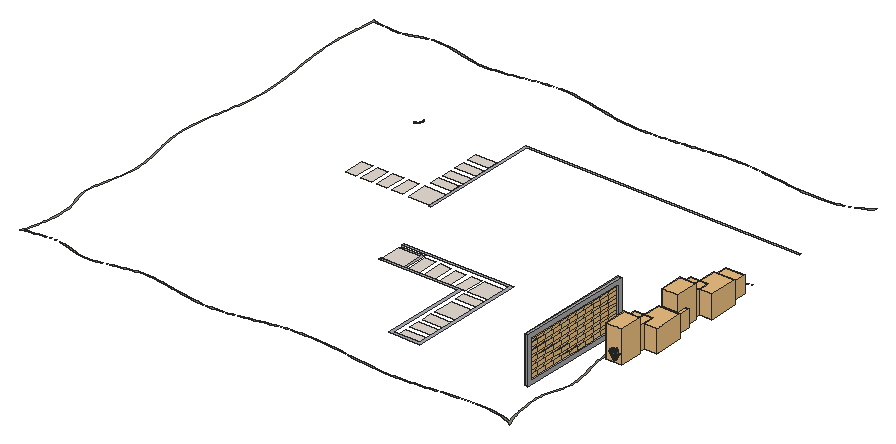
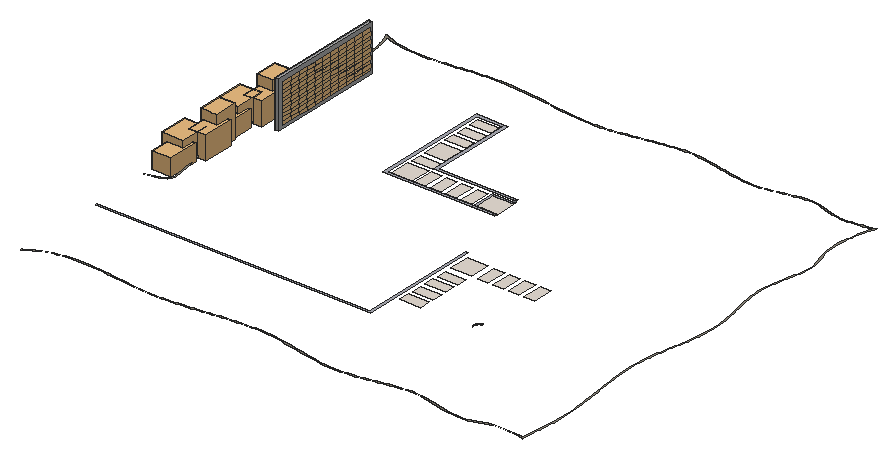
# SketchUp Ruby script. Lengths in inches.
U = 1.inch
M = Sketchup.active_model
def pt(a) = Geom::Point3d.new(a.map { |v| v * U })
def face(e, loops, mat)
  f = e.add_face(loops[0].map { |a| pt(a) })
  loops[1..].each { |l| e.add_face(l.map { |a| pt(a) }).erase! }
  f.material = f.back_material = mat if mat
  f
end
# faces: each face lists its corners as indices into pts; further lists are holes
def faces(e, pts, list, mat = nil) = list.each { |f| face(e, (f[0].is_a?(Array) ? f : [f]).map { |l| l.map { |i| pts[i] } }, mat) }
# xy, xz, yz: faces in a plane at the given z, y or x. An outline is a flat list of corners, or four numbers for a rectangle; further outlines are holes
def ring(l) = l.size == 4 ? [[l[0], l[1]], [l[2], l[1]], [l[2], l[3]], [l[0], l[3]]] : l.each_slice(2).to_a
def flat(e, list, mat, &to3) = list.each { |f| face(e, (f[0].is_a?(Array) ? f : [f]).map { |l| ring(l).map { |u, v| to3.(u, v) } }, mat) }
def xy(e, z, list, mat = nil) = flat(e, list, mat) { |x, y| [x, y, z] }
def xz(e, y, list, mat = nil) = flat(e, list, mat) { |x, z| [x, y, z] }
def yz(e, x, list, mat = nil) = flat(e, list, mat) { |y, z| [x, y, z] }
def lines(e, pts, list) = list.each { |a, b| e.add_line(pt(pts[a]), pt(pts[b])) }
# prism: a flat outline (further loops are holes) pulled along v
def prism(e, loops, v, mat = nil)
  f = face(e, loops, mat); d = Geom::Vector3d.new(v.map { |x| x * U })
  f.pushpull(f.normal.samedirection?(d) ? d.length : -d.length)
end
def box(e, o, s, mat = nil) = prism(e, [[o, [o[0] + s[0], o[1], o[2]], [o[0] + s[0], o[1] + s[1], o[2]], [o[0], o[1] + s[1], o[2]]]], [0, 0, s[2]], mat)
def at(x, y, z, deg = 0) = Geom::Transformation.translation(pt([x, y, z])) * Geom::Transformation.rotation(ORIGIN, Z_AXIS, deg.degrees)
def axes(o, x, y, z) = Geom::Transformation.new([*x, 0, *y, 0, *z, 0, *pt(o).to_a, 1])
def part(name) = M.definitions.add(name)
# library, detail: a bought-in or finely detailed component or shape, given as its bounding box
def library(name, o, s) = part(name).tap { |d| box(d.entities, o, s) }
def detail(e, o, s) = box(e.add_group.entities, o, s)
def put(e, d, t, mat = nil) = e.add_instance(d, t).tap { |i| i.material = mat if mat }
def group(e, t, mat = nil) = e.add_group.tap { |g| g.transformation = t; g.material = mat if mat }.entities
root = M.entities
M.materials.add("M03_Pewter_Shine").color = [168, 168, 168]
M.materials.add("Marble_01_1K").color = [230, 221, 211]
M.materials.add("Marble_07_1K").color = [36, 34, 36]
M.materials.add("Marble_20_1K").color = [172, 173, 182]
M.materials.add("Material__4").color = [36, 36, 36]
M.materials.add("Material__6").color = [79, 108, 5]
M.materials.add("Plaster_06_1K").color = [141, 135, 122]
M.materials.add("calathea lutea").color = [121, 145, 80]
c1 = library("Group\#103",[-0.1,0,0],[4.88,24.05,8.12])
c2 = part("Timber rail")
put(c2.entities,c1,axes([5.13,208.76,0],[-1,0,0],[0,-0.96445,0],[0,0,1]))
put(c2.entities,c1,axes([4.82,46.39,0],[-1,0,0],[0,-0.96445,0],[0,0,1]))
put(c2.entities,c1,axes([5,139.17,0],[-1,0,0],[0,-0.96445,0],[0,0,1]))
put(c2.entities,c1,axes([5.09,185.5625,0],[-1,0,0],[0,-0.96445,0],[0,0,1]))
put(c2.entities,c1,axes([5.04,162.37,0],[-1,0,0],[0,-0.96445,0],[0,0,1]))
put(c2.entities,c1,axes([4.87,69.59,0],[-1,0,0],[0,-0.96445,0],[0,0,1]))
put(c2.entities,c1,axes([4.95,115.98,0],[-1,0,0],[0,-0.96445,0],[0,0,1]))
put(c2.entities,c1,axes([5.18,231.95,0],[-1,0,0],[0,-0.96445,0],[0,0,1]))
put(c2.entities,c1,axes([4.91,92.78,0],[-1,0,0],[0,-0.96445,0],[0,0,1]))
put(c2.entities,c1,axes([4.78,23.2,0],[-1,0,0],[0,-0.96445,0],[0,0,1]))
put(c2.entities,c1,axes([5.22,255.15,0],[-1,0,0],[0,-0.96445,0],[0,0,1]))
c3 = library("Group\#105",[0,0,0],[4.875,24.05,8.12])
c4 = part("Group\#104")
put(c4.entities,c3,axes([4.875,240.5,0],[-1,0,0],[0,1,0],[0,0,1]))
put(c4.entities,c3,axes([6.32,0,0],[-1,0,0],[0,1,0],[0,0,1]))
put(c4.entities,c3,axes([5.45,144.3,0],[-1,0,0],[0,1,0],[0,0,1]))
put(c4.entities,c3,axes([5.31,168.35,0],[-1,0,0],[0,1,0],[0,0,1]))
put(c4.entities,c3,axes([5.6,120.25,0],[-1,0,0],[0,1,0],[0,0,1]))
put(c4.entities,c3,axes([6.03,48.1,0],[-1,0,0],[0,1,0],[0,0,1]))
put(c4.entities,c3,axes([5.74,96.2,0],[-1,0,0],[0,1,0],[0,0,1]))
put(c4.entities,c3,axes([5.89,72.15,0],[-1,0,0],[0,1,0],[0,0,1]))
put(c4.entities,c3,axes([6.18,24.05,0],[-1,0,0],[0,1,0],[0,0,1]))
put(c4.entities,c3,axes([5.17,192.4,0],[-1,0,0],[0,1,0],[0,0,1]))
put(c4.entities,c3,axes([5.02,216.45,0],[-1,0,0],[0,1,0],[0,0,1]))
c5 = part("Group\#156")
g1 = group(c5.entities,at(8.61,38.85,0))
xy(g1,0,[[0,0,2.82,19.1,22.58,0],[22.58,0,2.82,19.1,22.58,19.1]],"calathea lutea")
p = [[2.82,19.1,0],[7.19,48.22,5.13],[10.77,48.22,5.13],[12.74,48.22,5.13],[22.58,48.22,5.13],[22.58,19.1,0]]
faces(g1,p,[[0,1,2,3,4,5]],"calathea lutea")
g2 = group(c5.entities,at(-0.77,-7.77,0))
p = [[14.8125,23.31,1.46],[21.35,23.31,0],[14.8125,0,1.46],[21.35,0,0],[27.89,0,1.46],[27.89,23.31,1.46],
  [8.27,46.62,2.92],[21.35,46.62,0],[34.4375,46.62,2.92],[4.47,23.31,6.43],[0,0,8.59],[33.76,0,4.28],
  [33.76,23.31,4.28]]
faces(g2,p,[[0,1,2],[3,2,1],[4,3,5],[1,5,3],[6,7,0],[1,0,7],[5,1,8],[7,8,1],
  [9,0,2,10],[11,4,5,12],[9,6,0],[12,5,8]],"calathea lutea")
c6 = part("Group\#150")
xy(c6.entities,0,[[0,0,0,33.87,27.21,33.87,19.71,0]],"calathea lutea")
c7 = part("Group\#157")
xy(c7.entities,1.04,[[21.13,33.87,21.13,57.59,32.375,57.59,27.12,33.87]],"calathea lutea")
xy(c7.entities,1.32,[[0.12,33.87,7.74,57.59]],"calathea lutea")
p = [[7.74,33.87,1.32],[11.8,57.59,0.61],[15.24,57.59,0],[15.24,33.87,0],[18.43,57.59,0.5625],[21.13,57.59,1.04],
  [21.13,33.87,1.04],[15.24,77.7,2.36],[21.13,77.7,3.4],[7.74,57.59,1.32],[7.74,77.7,3.69],[36.83,77.7,3.4],
  [32.375,57.59,1.04],[0.12,57.59,1.32],[0.12,77.7,3.69]]
faces(c7.entities,p,[[0,1,2,3],[3,2,4],[3,4,5,6],[7,2,1],[8,4,2,7],[0,9,1],[7,1,9,10],[8,5,4],
  [11,12,5,8],[10,9,13,14]],"calathea lutea")
put(c7.entities,c6,axes([0,-16.9375,0],[1,0,0],[0,1.5,0],[0,0,1]))
c8 = part("Group\#155")
g3 = group(c8.entities,at(0,-17.3,0))
xy(g3,0,[[0,0,28.07,51.9]],"calathea lutea")
g4 = group(c8.entities,at(0.9,34.6,0))
xy(g4,0,[[13.14,0,13.14,26.22,16.85,26.22],[13.14,0,16.85,26.22,20.16,26.22,20.16,0]],"calathea lutea")
p = [[6.36,0,1.82],[9.95,26.22,0.86],[13.14,26.22,0],[13.14,0,0],[20.16,0,0],[20.16,26.22,0],
  [27.07,26.22,1.22],[27.07,0,1.22],[13.14,49.5625,5.91],[20.16,49.5625,5.91],[16.85,26.22,0],[27.07,49.5625,7.125],
  [6.36,26.22,1.82],[6.36,49.5625,7.72],[0,0,4.78],[0,26.22,4.78],[0,49.5625,10.6875]]
faces(g4,p,[[0,1,2,3],[4,5,6,7],[8,2,1],[9,10,2,8],[9,5,10],[11,6,5,9],[0,12,1],[8,1,12,13],
  [14,15,12,0],[13,12,15,16]],"calathea lutea")
c9 = part("Group\#154")
put(c9.entities,c6,axes([0,-16.9375,0],[1,0,0],[0,1.5,0],[0,0,1]))
g5 = group(c9.entities,at(-0.23,33.4,-0.35))
p = [[15.12,39.14,-19.87],[15.12,20.54,-11.86],[11.68,20.84,-11.33],[21.02,39.66,-18.97],[18.3125,20.82,-11.37],[7.62,21.2,-10.71],
  [7.62,39.8,-18.72],[21.02,21.06,-10.96],[36.72,39.66,-18.97],[32.26,21.06,-10.96],[0,21.2,-10.71],[0,39.8,-18.72],
  [7.62,0.66,1.15],[15.12,0,0],[21.02,0.52,0.9],[27.01,0.52,0.9],[0,0.66,1.15]]
faces(g5,p,[[0,1,2],[3,4,1,0],[0,2,5,6],[3,7,4],[8,9,7,3],[6,5,10,11],[12,2,1,13],[13,1,4],
  [13,4,7,14],[12,5,2],[14,7,9,15],[16,10,5,12]],"calathea lutea")
c10 = part("Foliage cluster")
put(c10.entities,c5,axes([37.24,8.07,75.17],[1,0,0],[0,0.45554,-0.89021],[0,0.89021,0.45554]))
put(c10.entities,c7,axes([69.44,65.48,16.68],[-0.53288,-0.84619,0],[0.14694,-0.09253,0.98481],[-0.83334,0.52478,0.17365]))
put(c10.entities,c8,axes([47.9375,70.43,17.04],[0.74664,-0.66523,0],[0.11552,0.12965,0.98481],[-0.65512,-0.7353,0.17365]))
put(c10.entities,c5,axes([76.19,10.66,75.17],[0.70711,0.70711,0],[-0.32212,0.32212,-0.89021],[-0.62948,0.62948,0.45554]))
put(c10.entities,c5,axes([101.91,40.03,75.17],[0,1,0],[-0.45554,0,-0.89021],[-0.89021,0,0.45554]))
put(c10.entities,c5,axes([99.32,78.99,75.17],[-0.70711,0.70711,0],[-0.32212,-0.32212,-0.89021],[-0.62948,-0.62948,0.45554]))
put(c10.entities,c8,axes([34.81,63.36,17.04],[0.99956,-0.02967,0],[0.00515,0.17357,0.98481],[-0.02922,-0.98437,0.17365]))
put(c10.entities,c8,axes([48,37.4,15.8],[-0.14436,0.98953,0],[-0.40248,-0.05871,0.91355],[0.90398,0.13188,0.40674]))
put(c10.entities,c7,axes([56.87,39.77,12.28],[-0.67695,0.4263,0],[-0.18016,-0.28609,0.72505],[0.38636,0.61353,0.33809]))
put(c10.entities,c7,axes([36.12,43.25,12.28],[0.18947,0.77724,0],[-0.32848,0.08007,0.72505],[0.70442,-0.17172,0.33809]))
put(c10.entities,c9,axes([35.1,54.93,11.375],[0.79719,0.06694,0],[-0.03636,0.43302,0.6717],[0.05621,-0.66934,0.43454]))
put(c10.entities,c7,axes([41.66,47.32,12.28],[0.45082,0.66088,0],[-0.2793,0.19053,0.72505],[0.59896,-0.40858,0.33809]))
put(c10.entities,c7,axes([47.89,59.4,12.28],[0.79719,0.06694,0],[-0.02829,0.33691,0.72505],[0.06067,-0.7225,0.33809]))
put(c10.entities,c9,axes([29.53,49.96,11.375],[0.65692,0.45657,0],[-0.248,0.35682,0.6717],[0.38335,-0.55156,0.43454]))
put(c10.entities,c9,axes([29.9,49.27,12.86],[0.34062,0.72386,0],[-0.22849,0.10752,0.7591],[0.68685,-0.32321,0.25252]))
put(c10.entities,c9,axes([36.33,48.82,8.99],[0.09232,0.62522,0],[-0.3396,0.05015,0.53064],[0.52495,-0.07752,0.34329]))
put(c10.entities,c9,axes([49.82,38.52,8.99],[-0.54622,0.31791,0],[-0.17268,-0.29669,0.53064],[0.26692,0.45862,0.34329]))
put(c10.entities,c9,axes([55.68,39.21,8.99],[-0.632,0.00221,0],[-0.0012,-0.34328,0.53064],[0.00185,0.53064,0.34329]))
c11 = library("Group\#28",[0,0,0],[86.94,78.77,46.4375])
c12 = library("Group\#14",[-978.71,-103.24,719.12],[90.2,76.4,68.29])
c13 = library("Group\#13",[-906.16,-138.28,686.8],[98.25,106.18,75.79])
c14 = library("Group\#202",[-3.47,-2.45,12.47],[53.14,54.93,75.51])
c15 = part("Group\#33")
put(c15.entities,c10,axes([161.54,105.34,6.01],[0.19523,-0.19694,0],[0.19694,0.19523,0],[0,0,0.24957]))
put(c15.entities,c11,axes([0,77.52,0.92],[0.83,0,0],[0,0.83,0],[0,0,0.83]))
put(c15.entities,c12,axes([859.63,139.86,-568.1],[0.79,0,0],[0,0.79,0],[0,0,0.79]),"Material__4")
put(c15.entities,c13,axes([669.69,185.27,-472.48],[0.69,0,0],[0,0.69,0],[0,0,0.69]),"Material__6")
put(c15.entities,c14,at(132.78,74.93,-12.6))
xy(root,2,[[811.73,164.125,859.73,188.125],[811.73,200.125,859.73,224.125],[811.73,236.125,859.73,260.125],[811.73,272.27,859.73,320.125],[811.73,332.125,859.73,356.11],
  [613.51,368.125,661.51,415.98],[673.51,368.125,697.51,416.125],[709.51,368.125,733.51,416.125],[745.51,368.125,769.51,416.125],[781.51,368.125,805.51,416.125],
  [811.73,368.125,859.73,415.98],[360.08,576.64,384.08,624.64],[396.08,576.64,420.08,624.64],[432.08,576.64,456.08,624.64],[468.08,576.64,492.08,624.64],
  [506.43,576.78,554.43,624.64],[506.43,640.64,554.43,664.64],[506.43,676.64,554.43,700.64],[506.43,712.64,554.43,736.64],[506.43,748.64,554.43,772.64]],"Marble_01_1K")
xy(root,2,[[613.51,362.11,619.51,362.11,619.51,362.125,667.51,362.125,667.51,421.98,619.51,421.98,619.51,422.08,613.51,422.08,613.51,415.98,661.51,415.98,661.51,368.125,613.51,368.125]],"Marble_20_1K")
xy(root,6,[[797.8125,154.93,870.83,154.93,870.83,428.08,613.51,428.08,613.51,422.08,864.83,422.08,864.83,160.93,803.8125,160.93,803.8125,362.11,613.51,362.11,613.51,356.11,797.8125,356.11],[561.69,565.82,566.19,565.82,566.19,846.16,1202.44,846.16,1202.44,850.66,561.69,850.66]],"Marble_20_1K")
xy(root,6,[[480.86,22.51,492.06,22.83,503.17,23.57,514.21,24.67,525.18,26.08,536.08,27.75,546.93,29.625,557.72,31.65,568.47,33.79,579.18,35.98,589.86,38.16,600.5,40.3,611.13,42.34,621.74,44.22,632.34,45.9,642.93,47.33,653.53,48.46,664.15,49.25,674.79,49.72,685.46,49.9,696.15,49.8,706.86,49.47,717.6,48.91,728.36,48.17,739.13,47.25,749.92,46.2,760.72,45.03,771.53,43.77,782.36,42.45,793.19,41.09,804.03,39.72,814.875,38.36,825.72,37.04,836.57,35.79,847.42,34.64,858.27,33.6,869.12,32.71,879.96,31.99,890.79,31.46,901.62,31.17,912.43,31.12,923.23,31.35,934.02,31.83,944.82,32.55,955.63,33.45,966.5,34.5,977.4375,35.68,988.46,36.93,999.6,38.23,1010.87,39.55,1022.29,40.84,1033.89,42.07,1045.67,43.2,1057.57,44.17,1069.57,44.9,1081.6,45.34,1093.63,45.42,1105.61,45.08,1117.49,44.25,1129.23,42.86,1140.78,40.86,1152.09,38.1875,1163.13,34.77,1173.84,30.55,1184.2,25.47,1183.79,26.3125,1183.28,27.39,1179.64,35.07,1178.72,37.07,1177.76,39.51,1176.77,42.4,1175.76,45.76,1174.73,49.57,1173.6875,53.85,1172.63,58.59,1171.56,63.8,1170.47,69.48,1169.36,75.64,1168.22,82.24,1167.09,89.18,1166.03,96.4,1165.11,103.85,1164.36,111.45,1163.86,119.125,1163.64,126.82,1163.77,134.47,1164.3,142,1165.28,149.33,1166.75,156.44,1168.65,163.4,1170.82,170.26,1173.12,177.07,1175.38,183.88,1177.46,190.75,1179.17,197.72,1180.35,204.83,1180.94,212.02,1181.01,219.28,1180.625,226.6,1179.84,233.97,1178.73,241.39,1177.35,248.85,1175.76,256.35,1174.02,263.89,1172.2,271.46,1170.35,279.06,1168.54,286.68,1166.82,294.32,1165.24,301.97,1163.88,309.62,1162.78,317.27,1162.01,324.91,1161.58,332.57,1161.47,340.24,1161.66,347.9375,1162.11,355.64,1162.8,363.37,1163.7,371.1,1164.79,378.84,1166.02,386.58,1167.38,394.33,1168.83,402.07,1170.35,409.82,1171.91,417.56,1173.47,425.29,1175.01,433.01,1176.5,440.72,1177.9,448.42,1179.19,456.1,1180.35,463.77,1181.33,471.41,1182.11,479.04,1182.66,486.63,1182.96,494.19,1183.04,501.71,1182.91,509.1875,1182.59,516.63,1182.08,524.04,1181.41,531.41,1180.6,538.75,1179.65,546.06,1178.58,553.34,1177.41,560.59,1176.15,567.82,1174.82,575.03,1173.43,582.21,1172.01,589.375,1170.55,596.52,1169.09,603.65,1167.63,610.77,1166.2,617.87,1164.79,624.96,1163.4375,632.04,1162.15,639.12,1160.94,646.1875,1159.83,653.25,1158.82,660.32,1157.94,667.38,1157.2,674.44,1157.46,681.53,1162.47,688.71,1176.67,696.07,1204.46,703.68,1204.54,706.84,1175.31,699.43,1160.14,692.15,1154.57,684.97,1154.1,677.86,1154.79,670.79,1155.61,663.74,1156.54,656.72,1157.58,649.72,1158.71,642.73,1159.92,635.77,1161.19,628.82,1162.52,621.875,1163.88,614.95,1165.26,608.03,1166.66,601.11,1168.06,594.2,1169.44,587.29,1170.79,580.38,1172.11,573.46,1173.36,566.54,1174.55,559.61,1175.66,552.67,1176.67,545.72,1177.58,538.76,1178.36,531.78,1179.02,524.77,1179.52,517.75,1179.86,510.7,1180.03,503.63,1180.01,496.53,1179.79,489.4,1179.36,482.23,1178.71,475.04,1177.86,467.81,1176.85,460.55,1175.6875,453.26,1174.41,445.94,1173.04,438.6,1171.6,431.24,1170.12,423.86,1168.625,416.47,1167.14,409.05,1165.69,401.625,1164.31,394.18,1163.01,386.73,1161.82,379.28,1160.77,371.82,1159.89,364.35,1159.2,356.88,1158.72,349.42,1158.49,341.95,1158.52,334.5,1158.84,327.04,1159.49,319.6,1160.45,312.17,1161.67,304.76,1163.1,297.37,1164.7,290,1166.4,282.67,1168.16,275.37,1169.93,268.11,1171.64,260.91,1173.26,253.75,1174.72,246.65,1175.98,239.61,1176.99,232.63,1177.68,225.73,1178.02,218.9,1177.94,212.16,1177.4,205.5,1176.35,198.92,1174.81,192.43,1172.9,185.97,1170.77,179.51,1168.57,172.99,1166.42,166.38,1164.47,159.64,1162.85,152.72,1161.69,145.59,1160.98,138.29,1160.66,130.875,1160.7,123.4,1161.03,115.93,1161.61,108.51,1162.39,101.2,1163.33,94.07,1164.37,87.17,1165.46,80.55,1166.56,74.28,1167.62,68.42,1168.66,62.97,1169.69,57.96,1170.72,53.37,1171.73,49.1875,1172.74,45.42,1173.73,42.06,1174.72,39.09,1175.69,36.53,1176.66,34.3,1177.625,32.13,1166.5,36.75,1155.03,40.48,1143.29,43.4,1131.3,45.59,1119.13,47.1,1106.83,48.02,1094.43,48.42,1082,48.35,1069.58,47.91,1057.21,47.15,1044.95,46.15,1032.85,44.98,1020.95,43.71,1009.24,42.38,997.7,41.03,986.31,39.7,975.04,38.43,963.87,37.25,952.78,36.21,941.75,35.33,930.75,34.66,919.76,34.24,908.76,34.11,897.74,34.25,886.7,34.64,875.64,35.26,864.58,36.07,853.5,37.05,842.41,38.17,831.31,39.41,820.21,40.73,809.1,42.1,797.98,43.5,786.87,44.91,775.76,46.28,764.65,47.6,753.55,48.83,742.45,49.95,731.36,50.9375,720.28,51.75,709.21,52.37,698.15,52.76,687.11,52.9,676.09,52.76,665.09,52.31,654.11,51.52,643.15,50.38,632.21,48.92,621.28,47.18,610.35,45.24,599.43,43.15,588.49,40.95,577.54,38.7,566.57,36.47,555.57,34.29,544.53,32.24,533.45,30.36,522.33,28.71,511.15,27.35,499.91,26.32,488.61,25.69,477.22,25.51,465.76,25.83,454.22,26.71,442.59,28.1,430.88,29.9,419.11,32.01,407.27,34.32,395.39,36.71,383.47,39.09,371.51,41.34,359.53,43.37,347.53,45.05,335.52,46.29,323.52,46.98,311.53,47.01,299.55,46.27,287.6,44.73,275.71,42.54,263.875,39.93,252.13,37.12,240.5,34.3125,229,31.73,217.65,29.59,206.47,28.12,195.48,27.51,184.7,28,174.14,29.78,163.75,32.68,153.33,36.15,142.71,39.61,131.72,42.47,120.22,44.23,108.34,44.89,96.32,44.66,84.39,43.75,72.8,42.34,61.79,40.65,51.57,38.89,41.67,37.13,43.09,40.39,44.54,44.33,46,49.13,47.49,54.8125,48.99,61.4,50.52,68.9,52.08,77.33,53.7,86.63,55.27,96.65,56.63,107.19,57.64,118.07,58.12,129.1,57.92,140.1,56.89,150.88,54.875,161.27,52.04,171.24,48.82,180.9375,45.66,190.49,43.02,200.04,41.33,209.72,40.74,219.59,41.1,229.64,42.24,239.85,44,250.22,46.21,260.72,48.7,271.34,51.3,282.06,53.86,292.86,56.18,303.74,58.125,314.67,59.51,325.64,60.21,336.63,60.26,347.64,59.73,358.66,58.73,369.68,57.3125,380.7,55.58,391.71,53.61,402.7,51.48,413.66,49.28,424.6,47.09,435.5,45,446.36,43.08,457.16,41.42,467.91,40.1,478.6,39.2,489.21,38.78,499.75,38.79,510.22,39.2,520.63,39.97,530.98,41.04,541.28,42.39,551.52,43.96,561.72,45.72,571.88,47.61,582.01,49.61,592.11,51.66,602.1875,53.72,612.24,55.76,622.29,57.72,632.32,59.56,642.35,61.25,652.38,62.74,662.42,63.99,672.47,64.95,682.54,65.62,692.62,66,702.73,66.125,712.84,66.01,722.98,65.68,733.125,65.16,743.28,64.47,753.45,63.62,763.63,62.65,773.82,61.57,784.01,60.41,794.21,59.18,804.41,57.91,814.61,55.33,835.01,54.07,845.21,52.85,855.41,51.7,865.6,50.64,875.78,49.68,885.95,48.86,896.12,48.2,906.28,47.7,916.42,47.41,926.55,47.33,936.66,47.5,946.76,47.9,956.85,48.5,966.95,49.29,977.07,50.22,987.24,51.27,997.47,52.41,1007.78,53.62,1018.1875,54.85,1028.71,56.08,1039.36,67.2,1037.64,78.66,1036.06,90.58,1034.86,102.72,1034.28,114.82,1034.5,126.65,1035.76,137.99,1038.2,148.86,1041.51,159.45,1045.08,169.95,1048.32,180.54,1050.63,191.35,1051.61,202.38,1051.38,213.61,1050.19,225.03,1048.23,236.61,1045.76,248.33,1042.97,260.16,1040.1,272.1,1037.38,284.11,1035.02,296.17,1033.25,308.27,1032.27,320.39,1032.11,332.53,1032.64,344.66,1033.77,356.79,1035.38,368.91,1037.36,381.01,1039.59,393.07,1041.98,405.09,1044.41,417.0625,1046.76,428.97,1048.93,440.82,1050.8125,452.59,1052.29,464.27,1053.25,475.87,1053.64,487.38,1053.51,498.82,1052.92,510.1875,1051.92,521.49,1050.5625,532.74,1048.91,543.94,1047.03,555.1,1044.96,566.22,1042.77,577.32,1040.51,588.39,1038.24,599.44,1036.01,610.49,1033.89,621.54,1031.93,632.59,1030.19,643.65,1028.72,654.73,1027.59,665.83,1026.8125,676.95,1026.38,688.1,1026.27,699.26,1026.43,710.43,1026.85,721.625,1027.5,732.83,1028.35,744.04,1029.36,755.26,1030.51,766.49,1031.78,777.72,1033.12,788.95,1034.52,800.1875,1035.9375,811.42,1037.35,822.65,1038.73,833.875,1040.05,845.09,1041.27,856.3,1042.37,867.5,1043.32,878.68,1044.1,889.85,1044.66,901.01,1044.99,912.14,1045.04,923.26,1044.8125,934.37,1044.3,945.5,1043.55,956.67,1042.61,967.9,1041.5,979.23,1040.27,990.67,1038.95,1002.24,1037.6,1013.97,1036.24,1025.89,1034.91,1038.01,1033.66,1050.3125,1032.55,1062.76,1031.64,1075.29,1031.01,1087.86,1030.73,1100.42,1030.875,1112.91,1031.52,1125.29,1032.74,1137.5,1034.61,1149.5,1037.2,1161.22,1040.58,1172.64,1044.83,1183.68,1050.02,1194.31,1056.22,1204.46,1063.52,1204.46,1067.35,1194.96,1060.26,1185.03,1054.16,1174.69,1048.99,1163.99,1044.7,1152.96,1041.21,1141.65,1038.48,1130.1,1036.43,1118.36,1035,1106.47,1034.125,1094.48,1033.75,1082.43,1033.8,1070.375,1034.22,1058.36,1034.9375,1046.43,1035.89,1034.625,1037.02,1023,1038.25,1011.54,1039.54,1000.25,1040.85,989.09,1042.16,978.04,1043.42,967.08,1044.6,956.2,1045.66,945.36,1046.57,934.55,1047.3,923.74,1047.8,912.93,1048.04,902.09,1048,891.25,1047.72,880.4,1047.2,869.55,1046.49,858.68,1045.6,847.82,1044.57,836.95,1043.41,826.09,1042.16,815.22,1040.85,804.36,1039.49,793.5,1038.11,782.65,1036.75,771.8125,1035.43,760.98,1034.16,750.16,1032.99,739.36,1031.93,728.57,1031.01,717.79,1030.26,707.04,1029.7,696.31,1029.36,685.6,1029.27,674.92,1029.4375,664.26,1029.91,653.625,1030.7,643.01,1031.82,632.4,1033.25,621.78,1034.93,611.16,1036.82,600.52,1038.86,589.85,1041,579.16,1043.19,568.4375,1045.38,557.67,1047.52,546.86,1049.55,536,1051.43,525.07,1053.1,514.09,1054.51,503.03,1055.6,491.9,1056.34,480.68,1056.65,469.38,1056.49,457.99,1055.8125,446.53,1054.61,435.03,1052.97,423.48,1051.01,411.91,1048.82,400.3,1046.5,388.68,1044.16,377.04,1041.89,365.4,1039.79,353.77,1037.97,342.15,1036.51,330.55,1035.52,318.99,1035.09,307.46,1035.31,295.97,1036.29,284.47,1038,272.98,1040.26,261.51,1042.87,250.08,1045.63,238.71,1048.35,227.42,1050.82,216.22,1052.83,205.125,1054.18,194.15,1054.65,183.31,1054.03,172.66,1052.12,162.3,1049.17,152.0625,1045.75,141.79,1042.41,131.3,1039.67,120.39,1037.97,109.05,1037.28,97.5,1037.44,85.98,1038.27,74.72,1039.59,63.94,1041.19,53.47,1042.89,52.375,1033.38,51.27,1023.97,50.18,1014.65,49.125,1005.4,48.12,996.22,47.19,987.1,46.36,978.01,45.64,968.96,45.06,959.92,44.63,950.88,44.39,941.84,44.34,932.78,44.47,923.72,44.77,914.64,45.23,905.57,45.83,896.49,46.55,887.4,47.375,878.32,48.29,869.23,49.29,860.14,50.34,851.05,51.45,841.96,52.58,832.88,53.73,823.8,54.87,814.72,56,805.65,57.1,796.58,58.16,787.52,59.15,778.47,60.07,769.43,60.89,760.4,61.61,751.38,62.21,742.37,62.67,733.375,62.98,724.4,63.12,715.44,63.07,706.49,62.84,697.5625,62.39,688.65,61.71,679.76,60.79,670.88,59.66,662.01,58.34,653.13,56.85,644.25,55.24,635.36,53.52,626.45,51.74,617.54,49.91,608.6,48.07,599.64,46.26,590.66,44.49,581.64,42.8,572.6,41.22,563.51,39.78,554.39,38.51,545.22,37.4375,536.01,36.6,526.74,36.03,517.42,35.75,508.04,35.8,498.61,36.2,489.1,36.98,479.55,38.11,469.95,39.52,460.32,41.16,450.67,42.96,440.99,44.87,431.29,46.83,421.58,48.78,411.85,50.66,402.12,52.42,392.38,53.99,382.65,55.33,372.93,56.36,363.22,57.04,353.52,57.31,343.85,57.11,334.21,56.39,324.6,55.14,314.99,53.45,305.375,51.43,295.76,49.21,286.18,46.9,276.62,44.61,267.1,42.46,257.64,40.58,248.23,39.08,238.9,38.09,229.64,37.73,220.46,38.14,211.375,39.4375,202.41,41.59,193.65,44.27,185.04,47.16,176.49,49.9375,167.89,52.3,159.14,53.96,150.125,54.88,140.77,55.14,131.18,54.85,121.51,54.11,111.88,53.03,102.4375,51.73,93.31,50.3125,84.62,48.88,76.51,47.51,69.13,46.16,62.5,44.84,56.61,43.53,51.45,42.25,47.02,41,43.32,39.81,40.34,38.66,37.9,37.51,35.49,36.37,33.08,45.35,34.71,54.59,36.375,64.7,38.09,75.5,39.68,86.77,40.96,98.28,41.75,109.81,41.86,121.11,41.12,131.97,39.34,142.43,36.56,152.68,33.2,162.9,29.8,173.26,26.9,183.9,25.07,194.74,24.51,205.71,25.03,216.79,26.42,227.98,28.46,239.25,30.9375,250.61,33.66,262.02,36.42,273.48,39.01,284.95,41.24,296.43,42.92,307.9,43.87,319.41,44.07,330.96,43.62,342.54,42.61,354.15,41.14,365.76,39.31,377.38,37.21,389,34.9375,400.61,32.6,412.19,30.29,423.75,28.1,435.28,26.15,446.76,24.53,458.2,23.33,469.58,22.66]],"Plaster_06_1K")
xz(root,362.11,[[613.51,2,619.51,6]],"Marble_20_1K")
xz(root,422.08,[[613.51,2,619.51,6]],"Marble_20_1K")
yz(root,371.24,[[788.6875,18,788.75,19]],"Marble_07_1K")
yz(root,371.27,[[788.43,18,788.49,19]],"Marble_07_1K")
yz(root,371.28,[[788.23,18,788.3,19],[788.3,18,788.36,19]],"Marble_07_1K")
yz(root,371.29,[[787.78,18,787.88,19],[787.88,18,787.96,19],[787.96,18,788.04,19],[788.04,18,788.1,19],[788.1,18,788.17,19]],"Marble_07_1K")
p = [[359.76,775.25,18],[359.9375,775.26,18],[359.9375,775.26,19],[359.76,775.25,19],[360.14,775.27,18],[360.14,775.27,19],
  [360.36,775.29,18],[360.36,775.29,19],[360.6,775.31,18],[360.6,775.31,19],[360.85,775.33,18],[360.85,775.33,19],
  [361.12,775.36,18],[361.12,775.36,19],[361.39,775.39,18],[361.39,775.39,19],[361.67,775.43,18],[361.67,775.43,19],
  [361.96,775.48,18],[361.96,775.48,19],[362.24,775.53,18],[362.24,775.53,19],[362.52,775.59,18],[362.52,775.59,19],
  [362.8,775.66,18],[362.8,775.66,19],[363.08,775.74,18],[363.08,775.74,19],[363.35,775.82,18],[363.35,775.82,19],
  [363.625,775.91,18],[363.625,775.91,19],[363.9,776.01,18],[363.9,776.01,19],[364.17,776.11,18],[364.17,776.11,19],
  [364.4375,776.22,18],[364.4375,776.22,19],[364.7,776.34,18],[364.7,776.34,19],[364.96,776.46,18],[364.96,776.46,19],
  [365.22,776.59,18],[365.22,776.59,19],[365.48,776.73,18],[365.48,776.73,19],[365.73,776.875,18],[365.73,776.875,19],
  [365.98,777.02,18],[365.98,777.02,19],[366.22,777.18,18],[366.22,777.18,19],[366.46,777.35,18],[366.46,777.35,19],
  [366.7,777.52,18],[366.7,777.52,19],[366.9375,777.7,18],[366.9375,777.7,19],[367.17,777.9,18],[367.17,777.9,19],
  [367.41,778.11,18],[367.41,778.11,19],[367.64,778.35,18],[367.64,778.35,19],[367.875,778.6,18],[367.875,778.6,19],
  [368.11,778.875,18],[368.11,778.875,19],[368.35,779.18,18],[368.35,779.18,19],[368.59,779.52,18],[368.59,779.52,19],
  [368.85,779.9,18],[368.85,779.9,19],[369.11,780.34,18],[369.11,780.34,19],[369.4,780.85,18],[369.4,780.85,19],
  [369.7,781.4375,18],[369.7,781.4375,19],[370.02,782.11,18],[370.02,782.11,19],[370.37,782.88,18],[370.37,782.88,19],
  [370.59,783.7,18],[370.59,783.7,19],[370.76,784.42,18],[370.76,784.42,19],[370.9,785.05,18],[370.9,785.05,19],
  [371.01,785.59,18],[371.01,785.59,19],[371.09,786.06,18],[371.09,786.06,19],[371.15,786.45,18],[371.15,786.45,19],
  [371.19,786.79,18],[371.19,786.79,19],[371.22,787.07,18],[371.22,787.07,19],[371.25,787.3,18],[371.25,787.3,19],
  [371.26,787.49,18],[371.26,787.49,19],[371.28,787.65,18],[371.28,787.65,19],[371.29,787.78,18],[371.29,787.78,19],
  [371.29,788.17,18],[371.28,788.23,18],[371.28,788.23,19],[371.29,788.17,19],[371.28,788.36,18],[371.27,788.43,18],
  [371.27,788.43,19],[371.28,788.36,19],[371.27,788.49,18],[371.26,788.56,18],[371.26,788.56,19],[371.27,788.49,19],
  [371.25,788.62,18],[371.24,788.6875,18],[371.24,788.6875,19],[371.25,788.62,19],[371.24,788.75,18],[371.23,788.81,18],
  [371.23,788.81,19],[371.24,788.75,19],[371.22,788.88,18],[371.22,788.88,19],[371.21,788.94,18],[371.21,788.94,19],
  [371.2,789.01,18],[371.2,789.01,19],[371.18,789.07,18],[371.18,789.07,19],[371.17,789.13,18],[371.17,789.13,19],
  [371.16,789.2,18],[371.16,789.2,19],[371.14,789.26,18],[371.14,789.26,19],[371.13,789.32,18],[371.13,789.32,19],
  [371.12,789.39,18],[371.12,789.39,19],[371.1,789.45,18],[371.1,789.45,19],[371.08,789.51,18],[371.08,789.51,19],
  [371.07,789.58,18],[371.07,789.58,19],[371.05,789.64,18],[371.05,789.64,19],[371.03,789.7,18],[371.03,789.7,19],
  [371.01,789.76,18],[371.01,789.76,19],[370.99,789.83,18],[370.99,789.83,19],[370.97,789.89,18],[370.97,789.89,19],
  [370.95,789.95,18],[370.93,790.01,18],[370.93,790.01,19],[370.95,789.95,19],[370.91,790.07,18],[370.91,790.07,19],
  [370.89,790.13,18],[370.89,790.13,19],[370.86,790.19,18],[370.86,790.19,19],[370.84,790.25,18],[370.84,790.25,19],
  [370.8125,790.3125,18],[370.8125,790.3125,19],[370.79,790.375,18],[370.79,790.375,19],[370.76,790.43,18],[370.74,790.49,18],
  [370.74,790.49,19],[370.76,790.43,19],[370.71,790.55,18],[370.71,790.55,19],[370.68,790.61,18],[370.68,790.61,19],
  [370.65,790.67,18],[370.65,790.67,19],[370.625,790.73,18],[370.625,790.73,19],[370.6,790.78,18],[370.6,790.78,19],
  [370.57,790.84,18],[370.54,790.9,18],[370.54,790.9,19],[370.57,790.84,19],[370.51,790.96,18],[370.51,790.96,19],
  [370.47,791.01,18],[370.44,791.07,18],[370.44,791.07,19],[370.47,791.01,19],[370.41,791.125,18],[370.41,791.125,19],
  [370.375,791.18,18],[370.375,791.18,19],[370.34,791.24,18],[370.34,791.24,19],[370.31,791.29,18],[370.31,791.29,19],
  [370.27,791.35,18],[370.24,791.4,18],[370.24,791.4,19],[370.27,791.35,19],[370.2,791.46,18],[370.2,791.46,19],
  [370.16,791.51,18],[370.125,791.5625,18],[370.125,791.5625,19],[370.16,791.51,19],[370.09,791.61,18],[370.09,791.61,19],
  [370.05,791.67,18],[370.05,791.67,19],[370.01,791.72,18],[370.01,791.72,19],[369.97,791.77,18],[369.97,791.77,19],
  [369.93,791.82,18],[369.93,791.82,19],[369.89,791.87,18],[369.89,791.87,19],[369.85,791.92,18],[369.81,791.97,18],
  [369.81,791.97,19],[369.85,791.92,19],[369.77,792.02,18],[369.73,792.07,18],[369.73,792.07,19],[369.77,792.02,19],
  [369.68,792.12,18],[369.64,792.17,18],[369.64,792.17,19],[369.68,792.12,19],[369.59,792.22,18],[369.59,792.22,19],
  [369.55,792.26,18],[369.55,792.26,19],[369.51,792.3125,18],[369.51,792.3125,19],[369.46,792.36,18],[369.46,792.36,19],
  [369.37,792.45,18],[369.32,792.49,18],[369.32,792.49,19],[369.37,792.45,19],[369.41,792.4,18],[369.41,792.4,19],
  [359.87,775.87,18],[359.87,775.87,19],[360.23,775.9,18],[360.23,775.9,19],[360.59,775.93,18],[360.59,775.93,19],
  [360.96,775.97,18],[360.96,775.97,19],[361.31,776.01,18],[361.31,776.01,19],[361.66,776.06,18],[361.66,776.06,19],
  [361.99,776.11,18],[361.99,776.11,19],[362.3,776.18,18],[362.3,776.18,19],[362.6,776.24,18],[362.6,776.24,19],
  [362.89,776.32,18],[362.89,776.32,19],[363.16,776.39,18],[363.16,776.39,19],[363.43,776.48,18],[363.43,776.48,19],
  [363.69,776.57,18],[363.69,776.57,19],[363.95,776.67,18],[363.95,776.67,19],[364.2,776.77,18],[364.2,776.77,19],
  [364.45,776.89,18],[364.45,776.89,19],[364.7,777,18],[364.7,777,19],[364.94,777.125,18],[364.94,777.125,19],
  [365.18,777.26,18],[365.18,777.26,19],[365.42,777.39,18],[365.42,777.39,19],[365.65,777.53,18],[365.65,777.53,19],
  [365.88,777.68,18],[365.88,777.68,19],[366.11,777.83,18],[366.11,777.83,19],[366.33,777.99,18],[366.33,777.99,19],
  [366.55,778.16,18],[366.55,778.16,19],[366.76,778.33,18],[366.76,778.33,19],[366.97,778.51,18],[366.97,778.51,19],
  [367.17,778.7,18],[367.17,778.7,19],[367.36,778.9,18],[367.36,778.9,19],[367.55,779.1,18],[367.55,779.1,19],
  [367.73,779.32,18],[367.73,779.32,19],[367.91,779.54,18],[367.91,779.54,19],[368.07,779.77,18],[368.07,779.77,19],
  [368.23,780,18],[368.23,780,19],[368.39,780.24,18],[368.39,780.24,19],[368.53,780.49,18],[368.53,780.49,19],
  [368.68,780.74,18],[368.68,780.74,19],[368.82,780.99,18],[368.82,780.99,19],[368.95,781.25,18],[368.95,781.25,19],
  [369.08,781.51,18],[369.08,781.51,19],[369.2,781.77,18],[369.2,781.77,19],[369.32,782.03,18],[369.32,782.03,19],
  [369.43,782.3,18],[369.43,782.3,19],[369.54,782.5625,18],[369.54,782.5625,19],[369.65,782.83,18],[369.65,782.83,19],
  [369.75,783.1,18],[369.75,783.1,19],[369.84,783.375,18],[369.84,783.375,19],[369.93,783.65,18],[369.93,783.65,19],
  [370.01,783.93,18],[370.01,783.93,19],[370.09,784.2,18],[370.09,784.2,19],[370.17,784.48,18],[370.17,784.48,19],
  [370.23,784.76,18],[370.23,784.76,19],[370.3,785.04,18],[370.3,785.04,19],[370.36,785.33,18],[370.36,785.33,19],
  [370.41,785.61,18],[370.41,785.61,19],[370.46,785.89,18],[370.46,785.89,19],[370.5,786.16,18],[370.5,786.16,19],
  [370.54,786.43,18],[370.54,786.43,19],[370.57,786.68,18],[370.57,786.68,19],[370.6,786.91,18],[370.6,786.91,19],
  [370.625,787.12,18],[370.625,787.12,19],[370.64,787.31,18],[370.64,787.31,19],[370.66,787.47,18],[370.66,787.47,19],
  [370.67,787.6,18],[370.67,787.6,19],[370.68,787.72,18],[370.68,787.72,19],[370.69,787.8125,18],[370.69,787.8125,19],
  [370.6875,787.89,18],[370.6875,787.89,19],[370.6875,787.96,18],[370.6875,787.96,19],[370.6875,788.02,18],[370.6875,788.02,19],
  [370.6875,788.08,18],[370.6875,788.08,19],[370.68,788.14,18],[370.68,788.14,19],[370.68,788.2,18],[370.68,788.2,19],
  [370.68,788.26,18],[370.68,788.26,19],[370.67,788.32,18],[370.67,788.32,19],[370.67,788.38,18],[370.67,788.38,19],
  [370.66,788.4375,18],[370.66,788.4375,19],[370.66,788.49,18],[370.66,788.49,19],[370.65,788.55,18],[370.65,788.55,19],
  [370.65,788.61,18],[370.65,788.61,19],[370.64,788.67,18],[370.64,788.67,19],[370.63,788.73,18],[370.63,788.73,19],
  [370.62,788.79,18],[370.62,788.79,19],[370.61,788.84,18],[370.61,788.84,19],[370.6,788.9,18],[370.6,788.9,19],
  [370.59,788.96,18],[370.59,788.96,19],[370.58,789.02,18],[370.58,789.02,19],[370.57,789.07,18],[370.57,789.07,19],
  [370.56,789.13,18],[370.56,789.13,19],[370.54,789.1875,18],[370.54,789.1875,19],[370.53,789.25,18],[370.53,789.25,19],
  [370.51,789.3,18],[370.51,789.3,19],[370.5,789.36,18],[370.5,789.36,19],[370.48,789.42,18],[370.48,789.42,19],
  [370.47,789.47,18],[370.47,789.47,19],[370.45,789.53,18],[370.45,789.53,19],[370.44,789.59,18],[370.44,789.59,19],
  [370.42,789.64,18],[370.42,789.64,19],[370.4,789.7,18],[370.4,789.7,19],[370.38,789.75,18],[370.38,789.75,19],
  [370.36,789.81,18],[370.36,789.81,19],[370.34,789.86,18],[370.34,789.86,19],[370.32,789.92,18],[370.32,789.92,19],
  [370.3,789.97,18],[370.3,789.97,19],[370.28,790.03,18],[370.28,790.03,19],[370.26,790.08,18],[370.26,790.08,19],
  [370.23,790.14,18],[370.23,790.14,19],[370.21,790.19,18],[370.21,790.19,19],[370.1875,790.25,18],[370.1875,790.25,19],
  [370.16,790.3,18],[370.16,790.3,19],[370.14,790.35,18],[370.14,790.35,19],[370.11,790.41,18],[370.11,790.41,19],
  [370.09,790.46,18],[370.09,790.46,19],[370.06,790.51,18],[370.06,790.51,19],[370.03,790.5625,18],[370.03,790.5625,19],
  [370.01,790.61,18],[370.01,790.61,19],[369.98,790.67,18],[369.98,790.67,19],[369.95,790.72,18],[369.95,790.72,19],
  [369.92,790.77,18],[369.92,790.77,19],[369.89,790.82,18],[369.89,790.82,19],[369.86,790.87,18],[369.86,790.87,19],
  [369.83,790.92,18],[369.83,790.92,19],[369.8,790.97,18],[369.8,790.97,19],[369.77,791.02,18],[369.77,791.02,19],
  [369.73,791.07,18],[369.73,791.07,19],[369.7,791.12,18],[369.7,791.12,19],[369.67,791.17,18],[369.67,791.17,19],
  [369.63,791.21,18],[369.63,791.21,19],[369.6,791.26,18],[369.6,791.26,19],[369.57,791.31,18],[369.57,791.31,19],
  [369.53,791.36,18],[369.53,791.36,19],[369.49,791.4,18],[369.49,791.4,19],[369.46,791.45,18],[369.46,791.45,19],
  [369.42,791.49,18],[369.42,791.49,19],[369.38,791.54,18],[369.38,791.54,19],[369.35,791.59,18],[369.35,791.59,19],
  [369.31,791.63,18],[369.31,791.63,19],[369.27,791.67,18],[369.27,791.67,19],[369.23,791.72,18],[369.23,791.72,19],
  [369.19,791.76,18],[369.19,791.76,19],[369.15,791.81,18],[369.15,791.81,19],[369.11,791.85,18],[369.11,791.85,19],
  [369.07,791.89,18],[369.07,791.89,19],[369.03,791.93,18],[369.03,791.93,19],[368.99,791.97,18],[368.99,791.97,19],
  [368.95,792.02,18],[368.95,792.02,19],[368.91,792.06,18],[368.91,792.06,19],[368.86,792.1,18],[368.86,792.1,19],
  [368.82,792.14,18],[368.82,792.14,19],[368.78,792.18,18],[368.78,792.18,19],[368.73,792.21,18],[368.73,792.21,19],
  [368.6875,792.25,18],[368.6875,792.25,19],[368.64,792.29,18],[368.64,792.29,19],[368.6,792.33,18],[368.6,792.33,19],
  [368.55,792.37,18],[368.55,792.37,19],[368.51,792.4,18],[368.51,792.4,19],[368.46,792.4375,18],[368.46,792.4375,19],
  [368.42,792.47,18],[368.42,792.47,19]]
faces(root,p,[[0,1,2,3],[1,4,5,2],[4,6,7,5],[6,8,9,7],[8,10,11,9],[10,12,13,11],[12,14,15,13],[14,16,17,15],
  [16,18,19,17],[18,20,21,19],[20,22,23,21],[22,24,25,23],[24,26,27,25],[26,28,29,27],[28,30,31,29],[30,32,33,31],
  [32,34,35,33],[34,36,37,35],[36,38,39,37],[38,40,41,39],[40,42,43,41],[42,44,45,43],[44,46,47,45],[46,48,49,47],
  [48,50,51,49],[50,52,53,51],[52,54,55,53],[54,56,57,55],[56,58,59,57],[58,60,61,59],[60,62,63,61],[62,64,65,63],
  [64,66,67,65],[66,68,69,67],[68,70,71,69],[70,72,73,71],[72,74,75,73],[74,76,77,75],[76,78,79,77],[78,80,81,79],
  [80,82,83,81],[82,84,85,83],[84,86,87,85],[86,88,89,87],[88,90,91,89],[90,92,93,91],[92,94,95,93],[94,96,97,95],
  [96,98,99,97],[98,100,101,99],[100,102,103,101],[102,104,105,103],[104,106,107,105],[108,109,110,111],[112,113,114,115],[116,117,118,119],
  [120,121,122,123],[117,120,123,118],[124,125,126,127],[125,128,129,126],[128,130,131,129],[130,132,133,131],[132,134,135,133],[134,136,137,135],
  [136,138,139,137],[138,140,141,139],[140,142,143,141],[142,144,145,143],[144,146,147,145],[146,148,149,147],[148,150,151,149],[150,152,153,151],
  [152,154,155,153],[154,156,157,155],[156,158,159,157],[158,160,161,159],[162,163,164,165],[160,162,165,161],[163,166,167,164],[166,168,169,167],
  [168,170,171,169],[170,172,173,171],[172,174,175,173],[174,176,177,175],[178,179,180,181],[176,178,181,177],[179,182,183,180],[182,184,185,183],
  [184,186,187,185],[186,188,189,187],[188,190,191,189],[192,193,194,195],[190,192,195,191],[193,196,197,194],[198,199,200,201],[196,198,201,197],
  [199,202,203,200],[202,204,205,203],[204,206,207,205],[206,208,209,207],[210,211,212,213],[208,210,213,209],[211,214,215,212],[216,217,218,219],
  [214,216,219,215],[217,220,221,218],[220,222,223,221],[222,224,225,223],[224,226,227,225],[226,228,229,227],[228,230,231,229],[232,233,234,235],
  [230,232,235,231],[236,237,238,239],[233,236,239,234],[240,241,242,243],[237,240,243,238],[241,244,245,242],[244,246,247,245],[246,248,249,247],
  [248,250,251,249],[252,253,254,255],[250,256,257,251],[256,252,255,257]],"Marble_07_1K")
lines(root,p,[[258,259],[260,261],[262,263],[264,265],[266,267],[268,269],[270,271],[272,273],[274,275],[276,277],[278,279],[280,281],
  [282,283],[284,285],[286,287],[288,289],[290,291],[292,293],[294,295],[296,297],[298,299],[300,301],[302,303],[304,305],
  [306,307],[308,309],[310,311],[312,313],[314,315],[316,317],[318,319],[320,321],[322,323],[324,325],[326,327],[328,329],
  [330,331],[332,333],[334,335],[336,337],[338,339],[340,341],[342,343],[344,345],[346,347],[348,349],[350,351],[352,353],
  [354,355],[356,357],[358,359],[360,361],[362,363],[364,365],[366,367],[368,369],[370,371],[372,373],[374,375],[376,377],
  [378,379],[380,381],[382,383],[384,385],[386,387],[388,389],[390,391],[392,393],[394,395],[396,397],[398,399],[400,401],
  [402,403],[404,405],[406,407],[408,409],[410,411],[412,413],[414,415],[416,417],[418,419],[420,421],[422,423],[424,425],
  [426,427],[428,429],[430,431],[432,433],[434,435],[436,437],[438,439],[440,441],[442,443],[444,445],[446,447],[448,449],
  [450,451],[452,453],[454,455],[456,457],[458,459],[460,461],[462,463],[464,465],[466,467],[468,469],[470,471],[472,473],
  [474,475],[476,477],[478,479],[480,481],[482,483],[484,485],[486,487],[488,489],[490,491],[492,493],[494,495],[496,497],
  [498,499],[500,501],[502,503],[504,505],[506,507],[508,509],[510,511],[512,513],[514,515],[516,517],[518,519],[520,521],
  [522,523],[524,525],[526,527],[528,529],[530,531],[532,533],[534,535],[536,537],[538,539],[540,541],[542,543],[544,545],
  [546,547],[548,549],[550,551],[552,553],[554,555],[556,557],[558,559],[560,561],[562,563],[564,565],[566,567],[568,569],
  [570,571]])
g6 = group(root,at(1113.83,154.93,6),"M03_Pewter_Shine")
prism(g6,[[[0,273.15,0],[0,0,0],[0,0,108],[0,273.15,108]],[[0,9,9],[0,264.15,9],[0,264.15,99],[0,9,99]]],[9,0,0])
g7 = group(root,at(1110.96,163.93,15))
put(g7,c2,axes([0,0,73.64],[1,0,0],[0,1,0],[0,0,1.01175]))
put(g7,c2,axes([0,0,57.29],[1,0,0],[0,1,0],[0,0,1.01175]))
put(g7,c2,axes([0,0,8.21],[1,0,0],[0,1,0],[0,0,1.01175]))
put(g7,c2,axes([0,0,24.57],[1,0,0],[0,1,0],[0,0,1.01175]))
put(g7,c2,axes([0,0,40.93],[1,0,0],[0,1,0],[0,0,1.01175]))
put(g7,c4,axes([0.49,0,81.79],[1,0,0],[0,0.96445,0],[0,0,1.01175]))
put(g7,c4,axes([0.49,0,65.43],[1,0,0],[0,0.96445,0],[0,0,1.01175]))
put(g7,c4,axes([0.49,0,49.07],[1,0,0],[0,0.96445,0],[0,0,1.01175]))
put(g7,c4,axes([0.49,0,16.36],[1,0,0],[0,0.96445,0],[0,0,1.01175]))
put(g7,c4,axes([0.49,0,32.71],[1,0,0],[0,0.96445,0],[0,0,1.01175]))
put(g7,c4,axes([0.49,0,0],[1,0,0],[0,0.96445,0],[0,0,1.01175]))
put(root,c15,axes([1113.16,515.28,0.74],[0,-1,0],[0.67442,0,0],[0,0,1]))
put(root,c15,axes([1113.16,677.09,0.74],[0,-1,0],[0.67442,0,0],[0,0,1]))
